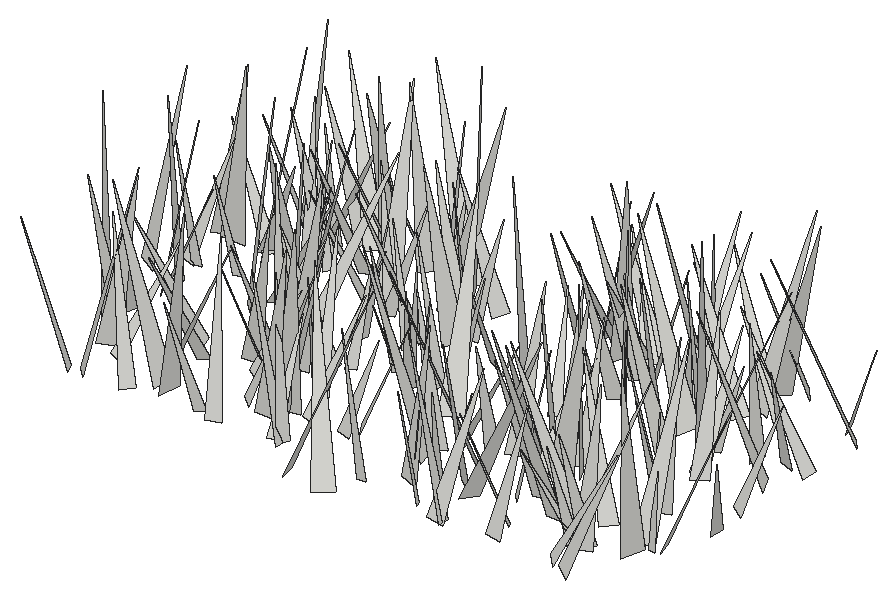
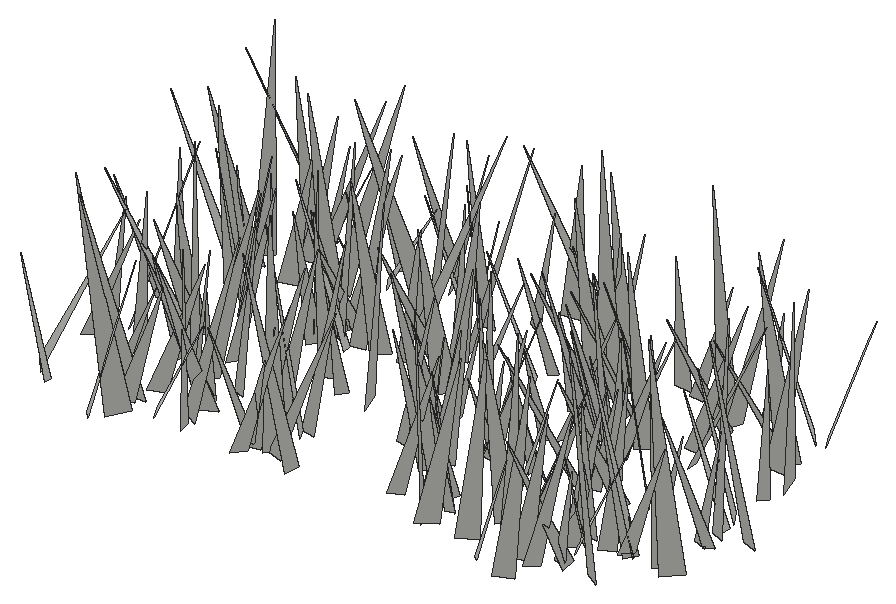
# SketchUp Ruby script. Lengths in inches.
U = 1.inch
M = Sketchup.active_model
def pt(a) = Geom::Point3d.new(a.map { |v| v * U })
def face(e, loops, mat)
  f = e.add_face(loops[0].map { |a| pt(a) })
  loops[1..].each { |l| e.add_face(l.map { |a| pt(a) }).erase! }
  f.material = f.back_material = mat if mat
  f
end
# faces: each face lists its corners as indices into pts; further lists are holes
def faces(e, pts, list, mat = nil) = list.each { |f| face(e, (f[0].is_a?(Array) ? f : [f]).map { |l| l.map { |i| pts[i] } }, mat) }
# xy, xz, yz: faces in a plane at the given z, y or x. An outline is a flat list of corners, or four numbers for a rectangle; further outlines are holes
def ring(l) = l.size == 4 ? [[l[0], l[1]], [l[2], l[1]], [l[2], l[3]], [l[0], l[3]]] : l.each_slice(2).to_a
def flat(e, list, mat, &to3) = list.each { |f| face(e, (f[0].is_a?(Array) ? f : [f]).map { |l| ring(l).map { |u, v| to3.(u, v) } }, mat) }
def xy(e, z, list, mat = nil) = flat(e, list, mat) { |x, y| [x, y, z] }
def xz(e, y, list, mat = nil) = flat(e, list, mat) { |x, z| [x, y, z] }
def yz(e, x, list, mat = nil) = flat(e, list, mat) { |y, z| [x, y, z] }
def lines(e, pts, list) = list.each { |a, b| e.add_line(pt(pts[a]), pt(pts[b])) }
# prism: a flat outline (further loops are holes) pulled along v
def prism(e, loops, v, mat = nil)
  f = face(e, loops, mat); d = Geom::Vector3d.new(v.map { |x| x * U })
  f.pushpull(f.normal.samedirection?(d) ? d.length : -d.length)
end
def box(e, o, s, mat = nil) = prism(e, [[o, [o[0] + s[0], o[1], o[2]], [o[0] + s[0], o[1] + s[1], o[2]], [o[0], o[1] + s[1], o[2]]]], [0, 0, s[2]], mat)
def at(x, y, z, deg = 0) = Geom::Transformation.translation(pt([x, y, z])) * Geom::Transformation.rotation(ORIGIN, Z_AXIS, deg.degrees)
def axes(o, x, y, z) = Geom::Transformation.new([*x, 0, *y, 0, *z, 0, *pt(o).to_a, 1])
def part(name) = M.definitions.add(name)
# library, detail: a bought-in or finely detailed component or shape, given as its bounding box
def library(name, o, s) = part(name).tap { |d| box(d.entities, o, s) }
def detail(e, o, s) = box(e.add_group.entities, o, s)
def put(e, d, t, mat = nil) = e.add_instance(d, t).tap { |i| i.material = mat if mat }
def group(e, t, mat = nil) = e.add_group.tap { |g| g.transformation = t; g.material = mat if mat }.entities
root = M.entities
c1 = part("fur_instance\#9")
p = [[0.8125,0,1.79],[0.67,-0.02,1.48],[0,-0.11,0],[0,0.11,0]]
faces(c1.entities,p,[[0,1,2,3]])
put(root,c1,axes([525.83,104.71,-21.66],[-2.86004,7.00076,0.77945],[7.00763,2.7424,1.08181],[-0.71502,-1.12544,7.48466]))
put(root,c1,axes([522.47,105.28,-21.66],[7.12948,2.21776,0.41944],[2.17259,-7.11974,0.71624],[-0.61174,0.56098,7.43203]))
put(root,c1,axes([503.1,107.16,-21.66],[-4.74174,-2.50609,0.51828],[-2.55748,4.67952,-0.77105],[0.09149,0.92453,5.30754]))
put(root,c1,axes([533.8125,106.15,-21.66],[0.03547,5.69131,1.501],[5.73382,0.30561,-1.29426],[1.32938,-1.46999,5.5423]))
put(root,c1,axes([534.32,106.38,-21.66],[-6.24639,-1.28271,0.8155],[-1.43317,6.11916,-1.35263],[0.50635,1.49608,6.23162]))
put(root,c1,axes([513.14,108.02,-21.66],[0.25989,-4.12749,1.06746],[-4.12688,-0.51192,-0.97467],[-1.06982,0.97209,4.01917]))
put(root,c1,axes([538.07,106.8,-21.66],[0.29151,4.89673,1.62599],[5.06271,0.04273,-1.03633],[0.99541,-1.65136,4.79468]))
put(root,c1,axes([542.84,106.84,-21.66],[3.55975,3.91646,0.08522],[3.79537,-3.41954,-1.38552],[0.97011,-0.99289,5.10792]))
put(root,c1,axes([531.6,107.22,-21.66],[-3.37291,-1.64413,0.77782],[-1.79286,3.28135,-0.83849],[0.30629,1.10194,3.65741]))
put(root,c1,axes([509.95,108.84,-21.66],[7.47084,-2.00529,1.5784],[-1.88161,-7.62701,-0.78379],[-1.72397,-0.36551,7.69548]))
put(root,c1,axes([544.35,106.04,-21.66],[4.64022,6.0526,0.40907],[6.0581,-4.59639,-0.71102],[0.31728,-0.75645,7.59342]))
put(root,c1,axes([526.85,107.35,-21.66],[-2.00481,-4.221,2.16779],[-4.72189,1.54205,-1.3643],[-0.46899,2.51807,4.46932]))
put(root,c1,axes([542.77,109.58,-21.66],[-3.89152,-1.38284,0.09587],[-1.31779,3.77936,1.02238],[0.42995,-0.93252,4.00136]))
put(root,c1,axes([543.67,109.5625,-21.66],[3.33283,-3.55166,1.19436],[-3.37517,-3.53973,-1.10774],[-1.62758,0.06765,4.74288]))
put(root,c1,axes([533.24,107.18,-21.66],[3.40494,2.47984,0.75094],[2.39973,-3.48584,0.63038],[-0.97714,0.08048,4.16483]))
put(root,c1,axes([542.47,109.48,-21.66],[-3.58815,0.95471,1.93369],[1.59157,3.70529,1.12394],[1.45517,-1.69849,3.5388]))
put(root,c1,axes([519.88,107.92,-21.66],[-5.84783,-0.54956,0.92386],[-0.66437,5.86496,-0.71656],[0.84507,0.80798,5.82972]))
put(root,c1,axes([537.84,108.75,-21.66],[-3.22375,-2.36609,0.00506],[-2.25529,3.0702,-1.21594],[-0.71558,0.9831,3.80952]))
put(root,c1,axes([529.29,109.17,-21.66],[-0.7765,-5.95979,2.50914],[-6.25232,1.3369,1.24057],[1.65027,2.26084,5.88073]))
put(root,c1,axes([509.01,109.41,-21.66],[-7.26017,0.65472,1.63239],[0.85,7.37598,0.82207],[1.53976,-0.9847,7.24313]))
put(root,c1,axes([507.7,107.36,-21.66],[-5.44212,1.96061,0.21811],[1.90755,5.39324,-0.88463],[0.50284,0.7598,5.71648]))
put(root,c1,axes([519.85,108.06,-21.66],[-5.54219,0.95074,1.40051],[0.80502,5.69802,-0.68242],[1.48905,0.4581,5.58158]))
put(root,c1,axes([514.65,107.5,-21.66],[-0.46142,6.00885,1.03301],[6.04976,0.32253,0.82618],[-0.75742,-1.08443,5.96964]))
put(root,c1,axes([543.51,109.09,-21.66],[3.4619,-5.09824,2.22403],[-5.52391,-3.4582,0.67108],[-0.65172,2.22978,6.12588]))
put(root,c1,axes([546.36,110.7,-21.66],[6.94101,-3.43299,1.84422],[-3.2352,-7.17632,-1.18245],[-2.17258,-0.28153,7.65277]))
put(root,c1,axes([516.83,110.11,-21.66],[2.07554,-6.96607,1.71735],[-7.11885,-1.77704,1.39545],[0.89291,2.02467,7.13349]))
put(root,c1,axes([532.55,110.9,-21.66],[-2.91514,-5.53327,1.42514],[-5.42873,3.18122,1.24695],[1.78243,0.63944,6.12864]))
put(root,c1,axes([530.92,110.16,-21.66],[3.87563,-0.57439,1.14349],[-0.32332,-3.96837,-0.89752],[-1.23813,-0.76168,3.81378]))
put(root,c1,axes([504.06,107.25,-21.66],[5.15399,5.0376,1.12923],[4.93282,-5.27609,1.02292],[-1.5231,-0.04087,7.13405]))
put(root,c1,axes([519.14,108.05,-21.66],[-2.23012,3.65012,0.738],[3.54975,2.34365,-0.86487],[1.12574,-0.15918,4.18913]))
put(root,c1,axes([539.7,111.2,-21.66],[-1.24664,-7.42641,1.30497],[-7.49381,1.07378,-1.04811],[-0.83512,1.45053,7.45702]))
put(root,c1,axes([542.29,110.39,-21.66],[-7.15146,0.58689,0.88826],[0.71619,7.11549,1.06478],[0.78773,-1.14116,7.09606]))
put(root,c1,axes([533.6,109.96,-21.66],[7.07032,-2.50038,0.22823],[-2.5064,-6.98854,1.08245],[0.14815,1.09629,7.42089]))
put(root,c1,axes([517.47,111.4375,-21.66],[3.37968,-7.43588,1.46776],[-7.57694,-3.27406,0.85991],[0.19143,1.6903,8.12251]))
put(root,c1,axes([503.16,111.08,-21.66],[4.2743,-5.66959,1.70794],[-5.91958,-4.14155,1.06631],[-0.14077,2.00854,7.01974]))
put(root,c1,axes([503.41,112.21,-21.66],[0.65749,-6.30029,1.7132],[-6.47052,-0.85883,-0.67511],[-0.87239,1.62165,6.29842]))
put(root,c1,axes([514.63,110.91,-21.66],[2.82445,3.52777,0.66946],[3.53756,-2.58781,-1.2883],[0.61561,-1.31488,4.33162]))
put(root,c1,axes([531.93,113.11,-21.66],[-4.63636,-6.55031,0.51962],[-6.56307,4.58532,-0.75728],[-0.32055,0.86066,7.9893]))
put(root,c1,axes([509.1,113.46,-21.66],[0.9036,-5.03288,0.01557],[-4.93923,-0.88981,-0.97923],[-0.96652,-0.158,5.01871]))
put(root,c1,axes([528.16,112.43,-21.66],[-7.66466,-1.90179,1.421],[-1.79066,7.78455,0.75987],[1.55871,-0.40873,7.86043]))
put(root,c1,axes([537.15,112.77,-21.66],[-0.33805,-5.61743,0.95415],[-5.65981,0.22074,-0.70569],[-0.6576,0.9879,5.58317]))
put(root,c1,axes([522.22,111.29,-21.66],[0.51441,-3.71167,1.78135],[-3.92489,0.09986,1.3415],[1.24297,1.85145,3.49879]))
put(root,c1,axes([504.625,110.06,-21.66],[1.15422,4.7345,0.08294],[4.6056,-1.10261,-1.15208],[1.10037,-0.35121,4.73502]))
put(root,c1,axes([508.52,110.51,-21.66],[4.79219,0.94532,0.41054],[0.81575,-4.67249,1.23678],[-0.62985,1.14081,4.72537]))
put(root,c1,axes([517.87,110.53,-21.66],[5.65388,1.0827,1.74004],[0.6959,-5.81697,1.3583],[-1.92762,1.07564,5.59407]))
put(root,c1,axes([527.24,112.375,-21.66],[4.80931,3.10321,2.02961],[3.46778,-4.94111,-0.66234],[-1.31293,-1.68352,5.68513]))
put(root,c1,axes([547.49,112.59,-21.66],[5.84375,1.80801,0.13219],[1.81029,-5.79638,-0.74876],[0.09603,-0.75425,6.07105]))
put(root,c1,axes([519.3,111.38,-21.66],[0.97735,4.73028,0.44464],[4.65378,-0.86171,-1.06216],[0.95682,-0.64061,4.71196]))
put(root,c1,axes([522.7,112.51,-21.66],[4.03846,2.29721,0.25382],[2.30928,-3.98992,-0.63131],[0.09403,-0.6739,4.60302]))
put(root,c1,axes([547.07,111.78,-21.66],[1.77865,4.09096,1.0407],[3.89915,-2.02489,1.29578],[-1.61729,-0.38272,4.26855]))
put(root,c1,axes([536.0625,111.66,-21.66],[3.62964,3.56201,0.97293],[3.43547,-3.75775,0.94107],[-1.35352,0.01415,4.99765]))
put(root,c1,axes([528.16,113.54,-21.66],[1.39978,-5.30319,2.32473],[-5.64349,-1.78474,-0.67328],[-1.29585,2.04412,5.44334]))
put(root,c1,axes([542.875,112.61,-21.66],[-3.19469,4.99874,1.10839],[5.10889,3.02549,1.08057],[-0.33936,-1.5103,5.83317]))
put(root,c1,axes([507.88,115.08,-21.66],[-5.4355,-1.48683,0.1699],[-1.41481,5.31415,1.24191],[0.48767,-1.15472,5.49664]))
put(root,c1,axes([534.19,116.32,-21.66],[-0.43827,-6.52973,0.002],[-6.42899,0.43186,1.145],[1.14256,-0.07472,6.44348]))
put(root,c1,axes([513.7,114.24,-21.66],[-2.53875,-3.10556,0.31926],[-3.0835,2.42999,-0.88252],[-0.48832,0.80145,3.91291]))
put(root,c1,axes([546.03,112.22,-21.66],[-1.91497,6.86191,1.78883],[6.91485,2.21764,-1.10438],[1.57179,-1.39609,7.03799]))
put(root,c1,axes([511.66,115.16,-21.66],[2.30675,-6.01681,0.97122],[-6.03702,-2.11321,1.24701],[0.83643,1.34116,6.32203]))
put(root,c1,axes([515.02,112.92,-21.66],[4.28943,0.41298,0.87796],[0.18379,-4.25331,1.1028],[-0.95267,1.03894,4.16576]))
put(root,c1,axes([501.53,115.66,-21.66],[3.7269,-2.05729,0.24824],[-1.97365,-3.67974,-0.86491],[-0.63149,-0.64103,4.16823]))
put(root,c1,axes([501.33,113.27,-21.66],[-7.33304,-1.55705,2.53328],[-2.07568,7.50758,-1.39398],[2.1292,1.95633,7.36578]))
put(root,c1,axes([536.71,115.34,-21.66],[-1.94061,6.26278,4.61542],[7.19839,3.24975,-1.38302],[2.95087,-3.80883,6.40903]))
put(root,c1,axes([548.84,116.17,-21.66],[3.9114,-1.46291,0.01114],[-1.40736,-3.77134,-1.11157],[-0.39945,-1.03737,4.02536]))
put(root,c1,axes([516.36,115.63,-21.66],[2.79226,2.81825,2.22878],[3.51982,-2.71249,-0.9798],[-0.72174,-2.32521,3.84438]))
put(root,c1,axes([525.09,115.17,-21.66],[-2.96371,-3.18096,0.56073],[-3.21747,2.84043,-0.89238],[-0.28422,1.01488,4.25508]))
put(root,c1,axes([530.68,115.92,-21.66],[2.96444,-3.24193,0.90441],[-3.19075,-3.09049,-0.61962],[-1.07107,0.23387,4.34903]))
put(root,c1,axes([512.91,113.75,-21.66],[2.64419,5.03318,0.33977],[4.95036,-2.51506,-1.26831],[0.97076,-0.88412,5.54221]))
put(root,c1,axes([514.43,116.13,-21.66],[3.42079,-7.2545,1.9343],[-7.49487,-3.17419,1.34998],[0.44283,2.31686,7.90614]))
put(root,c1,axes([535.65,116.32,-21.66],[3.71105,4.69804,3.51461],[5.68502,-3.90755,-0.77947],[-1.45074,-3.29476,5.93598]))
put(root,c1,axes([529.1,114.6,-21.66],[4.45979,0.0367,0.09292],[0.01604,-4.35825,0.95137],[-0.0986,0.95079,4.35729]))
put(root,c1,axes([544.46,115.97,-21.66],[3.53738,-5.32848,1.99163],[-5.66565,-3.51029,0.67133],[-0.50966,2.039,6.36044]))
put(root,c1,axes([512.27,116.77,-21.66],[-0.63614,-4.28295,0.71253],[-4.25699,0.4736,-0.95381],[-0.85404,0.8295,4.22357]))
put(root,c1,axes([536.11,115.47,-21.66],[4.52049,-0.19473,1.20973],[-0.39564,-4.60837,0.73662],[-1.15967,0.81315,4.46432]))
put(root,c1,axes([535.64,114.41,-21.66],[-1.08496,4.24211,0.2137],[4.12597,1.10497,-0.98676],[1.00871,0.04308,4.26602]))
put(root,c1,axes([517.94,114.35,-21.66],[-0.8094,5.47668,0.09308],[5.43232,0.79056,0.72297],[-0.70181,-0.19701,5.48875]))
put(root,c1,axes([534.66,116.9,-21.66],[5.44749,2.02001,0.26599],[2.02291,-5.27178,-1.39377],[0.24298,-1.39796,5.64031]))
put(root,c1,axes([542.72,117.6,-21.66],[3.69815,0.46024,1.83595],[1.02421,-3.87534,-1.09159],[-1.5917,-1.42435,3.56322]))
put(root,c1,axes([532.54,116.07,-21.66],[-2.8521,5.31504,2.52319],[5.50682,3.39878,-0.93481],[2.07151,-1.71732,5.95905]))
put(root,c1,axes([542.52,118.02,-21.66],[-4.88015,-2.78524,1.52655],[-2.68194,5.11285,0.7548],[1.7015,0.07051,5.5681]))
put(root,c1,axes([544.2,115.77,-21.66],[4.62309,3.63215,1.82021],[3.50208,-4.96051,1.00367],[-2.05939,-0.28182,5.79293]))
put(root,c1,axes([516.47,117.65,-21.66],[-5.33847,-0.05884,0.40473],[-0.0096,5.31499,0.64603],[0.40887,-0.64342,5.29956]))
put(root,c1,axes([521.91,118.4,-21.66],[4.60045,-1.39498,0.802],[-1.20201,-4.59424,-1.0961],[-1.06973,-0.83684,4.68067]))
put(root,c1,axes([537.4,116.625,-21.66],[-5.47988,-2.79163,2.54101],[-3.31815,5.69792,-0.89593],[1.79996,2.00489,6.08438]))
put(root,c1,axes([539.3,118.63,-21.66],[4.52719,2.71843,2.25301],[3.1828,-4.72799,-0.69084],[-1.52829,-1.79378,5.23527]))
put(root,c1,axes([513,117.35,-21.66],[-6.34859,-2.07949,3.15929],[-2.7531,6.77324,-1.07409],[2.59343,2.09974,6.59357]))
put(root,c1,axes([512.7,117.11,-21.66],[5.61181,2.09612,1.30854],[1.89864,-5.73587,1.04566],[-1.58152,0.55181,5.89854]))
put(root,c1,axes([536.69,117.59,-21.66],[3.58302,-2.92408,2.58959],[-3.63927,-3.77537,0.77237],[-1.41842,2.30013,4.5598]))
put(root,c1,axes([514.33,116.67,-21.66],[2.31766,5.02687,0.82298],[4.84651,-2.45447,1.34356],[-1.56781,-0.15629,5.3699]))
put(root,c1,axes([512.23,117.46,-21.66],[-5.96382,1.04535,0.88629],[0.82737,5.90096,-1.39268],[1.09259,1.23747,5.8924]))
put(root,c1,axes([517.27,118.26,-21.66],[-2.50227,2.59124,1.1484],[2.47228,2.74461,-0.80603],[1.38608,-0.21748,3.51087]))
put(root,c1,axes([521,119.76,-21.66],[-1.15878,-4.12917,1.68532],[-4.31214,1.48176,0.66553],[1.13832,1.40977,4.23673]))
put(root,c1,axes([548.17,119.15,-21.66],[1.81296,4.05322,0.9149],[4.0683,-1.5284,-1.29051],[0.84535,-1.3371,4.24853]))
put(root,c1,axes([519.85,119.73,-21.66],[-1.05409,-4.02831,1.60299],[-4.27873,0.70037,-1.05356],[-0.69957,1.78611,4.02845]))
put(root,c1,axes([526.15,117.43,-21.66],[-5.32969,5.59283,1.04722],[5.46672,5.43108,-1.18331],[1.57839,0.07463,7.63447]))
put(root,c1,axes([500.93,120.21,-21.66],[4.64757,1.11707,0.03174],[1.0994,-4.54603,-0.98676],[0.20042,-0.96672,4.67697]))
put(root,c1,axes([501.52,118.66,-21.66],[-4.45958,-2.36263,3.46386],[-3.3219,5.07642,-0.81428],[2.55838,2.47306,4.98064]))
put(root,c1,axes([500.88,121.2,-21.66],[-3.13728,-6.42445,2.27927],[-6.51063,3.56742,1.09378],[2.01998,1.52023,7.06539]))
put(root,c1,axes([533.22,120.59,-21.66],[1.79677,-5.19077,1.98742],[-5.55817,-1.66844,0.66734],[0.02536,2.09632,5.45226]))
put(root,c1,axes([512.23,119.02,-21.66],[7.1658,2.76652,1.69463],[2.58302,-7.35112,1.0785],[-1.96302,0.42601,7.60521]))
put(root,c1,axes([510.76,121.36,-21.66],[1.65267,-3.08975,1.39314],[-3.11179,-1.99748,-0.7386],[-1.34319,0.82596,3.42525]))
put(root,c1,axes([523.22,119.97,-21.66],[-5.0928,-0.09663,0.30052],[-0.16718,4.94609,-1.24277],[0.26777,1.25023,4.93978]))
put(root,c1,axes([547.4375,122.9375,-21.66],[-6.20771,-3.16783,0.82777],[-3.08728,6.25411,0.78157],[1.09042,-0.32718,6.92531]))
put(root,c1,axes([524.13,120.52,-21.66],[3.78689,-0.0231,1.24793],[-0.32688,-3.86581,0.92039],[-1.20458,0.97644,3.67342]))
put(root,c1,axes([498.52,120.87,-21.66],[3.30058,6.51639,2.13105],[6.85171,-3.21879,-0.76942],[-0.24255,-2.25268,7.26396]))
put(root,c1,axes([539.24,122.68,-21.66],[-6.05597,0.77226,2.0179],[1.21073,6.18666,1.26588],[1.78953,-1.57224,5.97233]))
put(root,c1,axes([507.14,120.44,-21.66],[4.85297,5.01471,2.08252],[4.89411,-5.24941,1.23566],[-2.35199,-0.5761,6.86817]))
put(root,c1,axes([529.1,121.48,-21.66],[-7.32615,-2.19993,2.60741],[-2.57876,7.61493,-0.82074],[2.23345,1.57604,7.60517]))
put(root,c1,axes([543.68,120.91,-21.66],[3.74309,-3.05687,3.19875],[-4.02453,-4.09315,0.7978],[-1.83838,2.73658,4.76642]))
put(root,c1,axes([514.06,122.37,-21.66],[2.61371,2.45973,0.53308],[2.49517,-2.43181,-1.01309],[0.32949,-1.09634,3.44317]))
put(root,c1,axes([524.23,124.29,-21.66],[-1.58112,-4.73276,0.31075],[-4.65779,1.61119,0.83937],[0.89473,0.02406,4.91878]))
put(root,c1,axes([515.36,121.86,-21.66],[4.20313,-0.16718,1.34956],[-0.39887,-4.34286,0.70427],[-1.30006,0.79192,4.14708]))
put(root,c1,axes([501.12,122.7,-21.66],[-0.94166,-4.10224,1.61468],[-4.38512,0.70145,-0.77524],[-0.45421,1.73259,4.13692]))
put(root,c1,axes([518.23,124.21,-21.66],[-5.1626,-2.88411,0.4563],[-2.82641,5.16852,0.6903],[0.7333,-0.3834,5.87316]))
put(root,c1,axes([507.92,122.01,-21.66],[4.70172,-1.10111,0.26171],[-1.12934,-4.49092,1.39405],[0.07438,1.41645,4.62334]))
put(root,c1,axes([503.99,123.31,-21.66],[-0.09942,-3.58739,1.13729],[-3.70553,-0.10534,-0.65623],[-0.65715,1.13676,3.52826]))
put(root,c1,axes([518.55,122.47,-21.66],[-0.54656,4.2534,1.19948],[4.32093,0.26075,1.04426],[-0.92722,-1.29209,4.15928]))
put(root,c1,axes([531.24,121.64,-21.66],[-2.96108,3.10315,0.36366],[3.04624,2.97875,-0.6142],[0.69442,0.16515,4.24503]))
put(root,c1,axes([543.19,121.43,-21.66],[-2.46279,4.53865,0.90199],[4.34757,2.61941,-1.3098],[1.58479,-0.13272,4.99491]))
put(root,c1,axes([500.37,122.74,-21.66],[0.61438,4.77457,1.24038],[4.786,-0.27399,-1.3159],[1.1955,-1.35681,4.63059]))
put(root,c1,axes([520.41,124.86,-21.66],[4.49335,-4.83843,2.48866],[-4.8443,-5.0271,-1.02712],[-2.47721,1.05444,6.5227]))
put(root,c1,axes([511.64,121.79,-21.66],[1.69788,6.23349,0.03172],[6.16311,-1.67374,-0.97718],[0.93461,-0.28707,6.38626]))
put(root,c1,axes([546.875,125.73,-21.66],[-0.66532,-4.77379,0.4836],[-4.67341,0.75535,1.0268],[1.0873,0.32553,4.70929]))
put(root,c1,axes([542.84,122.4,-21.66],[6.48449,2.8801,0.19854],[2.8437,-6.45643,0.78158],[-0.49773,0.63448,7.05214]))
put(root,c1,axes([536.36,125.76,-21.66],[-2.50316,-5.2047,1.47138],[-5.2002,2.76171,0.92225],[1.48721,0.89649,5.70124]))
put(root,c1,axes([532.87,125.8125,-21.66],[1.51569,-5.39227,1.25729],[-5.41404,-1.71643,-0.83467],[-1.15995,0.96539,5.5387]))
put(root,c1,axes([544.9375,125.22,-21.66],[-4.81176,0.83188,2.6308],[1.27412,5.3609,0.63523],[2.44739,-1.15538,4.84165]))
put(root,c1,axes([542.14,124.41,-21.66],[2.6099,-2.39325,0.8726],[-2.54736,-2.4537,0.88934],[-0.00348,1.24593,3.42758]))
put(root,c1,axes([512.07,126.12,-21.66],[-4.07436,-2.22938,0.28557],[-2.14023,4.02883,0.91657],[0.68639,-0.67121,4.55307]))
put(root,c1,axes([539.99,125.67,-21.66],[7.38345,1.68053,2.79244],[2.22073,-7.65548,-1.26461],[-2.38543,-1.92527,7.46594]))
put(root,c1,axes([548.79,125.73,-21.66],[-4.51725,1.3418,0.80765],[1.52463,4.33149,1.33117],[0.35811,-1.51528,4.52039]))
put(root,c1,axes([529.7,127.03,-21.66],[-1.86711,-6.21996,0.83765],[-6.21183,1.95621,0.67975],[0.89595,0.60083,6.45848]))
put(root,c1,axes([505.19,127.04,-21.66],[4.3108,-3.69492,0.61953],[-3.55093,-4.33068,-1.12044],[-1.19463,-0.46051,5.56597]))
put(root,c1,axes([539.13,125.43,-21.66],[-7.00283,2.97011,1.6591],[3.21934,7.01289,1.03394],[1.10002,-1.61605,7.53606]))
put(root,c1,axes([500.92,126.63,-21.66],[1.84601,-7.44066,1.73932],[-7.59322,-1.58595,1.27441],[0.85535,1.97933,7.55956]))
put(root,c1,axes([499.92,127.03,-21.66],[4.60789,-6.31495,1.14074],[-6.41656,-4.51508,0.92427],[0.08686,1.46561,7.76253]))
put(root,c1,axes([534.02,125.18,-21.66],[3.38997,4.6985,2.258],[4.82742,-3.84601,0.75539],[-1.96736,-1.34115,5.74432]))
put(root,c1,axes([514.75,125.18,-21.66],[3.82826,-1.89723,1.31218],[-2.241,-3.66166,1.2438],[-0.54703,1.72325,4.08754]))
put(root,c1,axes([503.53,126.77,-21.66],[3.31192,-3.28223,0.0309],[-3.2384,-3.26025,0.79144],[0.53549,0.5836,4.59516]))
put(root,c1,axes([520.81,126.02,-21.66],[1.98838,-4.24744,1.75797],[-4.57109,-1.62434,1.24561],[0.4862,2.09896,4.52138]))
put(root,c1,axes([520.7,125.84,-21.66],[-4.62696,-2.40171,1.71965],[-2.7299,4.69747,-0.78458],[1.12828,1.51649,5.15378]))
put(root,c1,axes([539.83,125.88,-21.66],[-4.89428,-1.48699,1.50253],[-1.73277,4.99254,-0.70337],[1.21087,1.13406,5.0666]))
put(root,c1,axes([537.2,127.65,-21.66],[0.94706,-3.59902,0.23008],[-3.53322,-0.8783,0.80484],[0.72266,0.42244,3.63347]))
put(root,c1,axes([519.43,126.89,-21.66],[-4.54367,3.48057,1.82928],[3.81076,4.58683,0.73803],[0.96889,-1.71821,5.67579]))
put(root,c1,axes([503.85,126.81,-21.66],[-3.48001,3.233,0.8636],[3.33945,3.27515,1.19585],[-0.21495,-1.45934,4.59703]))
put(root,c1,axes([529.92,127.42,-21.66],[6.22111,3.48137,1.76986],[3.77865,-6.20685,-1.07301],[-0.98698,-1.81924,7.04775]))
put(root,c1,axes([510.18,128.58,-21.66],[-0.32554,-5.06602,0.7464],[-4.99056,0.14633,-1.18345],[-1.14716,0.80105,4.9366]))
put(root,c1,axes([513.71,126.72,-21.66],[-0.78367,4.54033,1.31363],[4.69244,0.5877,0.76808],[-0.56674,-1.41222,4.54299]))
put(root,c1,axes([503.8,126.04,-21.66],[6.26441,4.08516,1.86388],[4.05019,-6.52197,0.68206],[-1.9387,-0.42509,7.44756]))
put(root,c1,axes([507.48,128.11,-21.66],[-4.95355,2.49117,1.9463],[2.93301,4.97148,1.10159],[1.17959,-1.90003,5.43416]))
put(root,c1,axes([507.28,126.39,-21.66],[-0.20928,5.81187,1.2771],[5.90875,0.05179,0.73257],[-0.70395,-1.2931,5.76932]))
put(root,c1,axes([532.45,128.65,-21.66],[0.82361,-5.861,1.93807],[-5.93962,-1.28507,-1.3621],[-1.68178,1.66825,5.75972]))
put(root,c1,axes([506.9,128.0625,-21.66],[-4.69197,-2.31538,0.05263],[-2.28134,4.60011,-1.00642],[-0.39908,0.92541,5.13447]))
put(root,c1,axes([508.08,127.42,-21.66],[-3.93894,0.78438,0.2139],[0.7314,3.88076,-0.76228],[0.35506,0.70765,3.94328]))
put(root,c1,axes([531.32,130.67,-21.66],[3.03189,-3.59681,0.02756],[-3.43565,-2.90654,-1.37057],[-1.06494,-0.8632,4.50011]))
put(root,c1,axes([510.91,130.9,-21.66],[-3.83453,-4.44323,0.31037],[-4.29048,3.7947,1.3169],[1.19597,-0.63261,5.71941]))
put(root,c1,axes([506.93,127.31,-21.66],[2.12896,3.50938,0.78952],[3.35263,-2.26833,1.04217],[-1.30344,-0.10245,3.97015]))
put(root,c1,axes([533.06,128.55,-21.66],[0.75971,3.71481,1.88794],[3.89435,-1.31575,1.02184],[-1.48263,-1.55251,3.65142]))
put(root,c1,axes([517.31,128.3125,-21.66],[7.2049,-3.47591,1.96261],[-3.83046,-7.15988,1.38131],[-1.1231,2.12096,7.87937]))
put(root,c1,axes([529.9,130.19,-21.66],[6.97183,-3.45055,1.53762],[-3.37643,-7.13932,-0.71191],[-1.69419,0.0288,7.74635]))
put(root,c1,axes([529.5,130.66,-21.66],[-1.20375,-5.21342,0.24756],[-5.17288,1.15789,-0.76855],[-0.69453,0.4118,5.2951]))
put(root,c1,axes([540.64,128.77,-21.66],[-4.45803,3.98436,0.74293],[4.03358,4.25341,1.39275],[-0.39655,-1.52789,5.81458]))
put(root,c1,axes([520.36,129.69,-21.66],[-4.35819,2.96505,1.59627],[3.3258,4.19926,1.28011],[0.52792,-1.97688,5.11338]))
put(root,c1,axes([512.49,128.2,-21.66],[-3.77046,5.93467,2.17976],[6.06315,4.1134,-0.71146],[1.79161,-1.43096,6.99504]))
put(root,c1,axes([536.93,130.14,-21.66],[-2.90211,-6.23156,1.67253],[-6.44447,2.71044,-1.08359],[-0.31368,1.96803,6.78825]))
put(root,c1,axes([543.29,129.8,-21.66],[-3.79672,1.89832,0.59417],[1.98792,3.66583,0.99077],[0.06937,-1.15319,4.1276]))
put(root,c1,axes([537.78,127.36,-21.66],[0.187,6.43803,0.46404],[6.40843,-0.12967,-0.78342],[0.77175,-0.48321,6.39292]))
put(root,c1,axes([516.23,129.34,-21.66],[0.00091,-3.67707,1.93886],[-4.08733,0.35251,0.67045],[0.75747,1.90654,3.61543]))
put(root,c1,axes([548.65,130.72,-21.66],[-5.4011,-4.4458,0.12135],[-4.40164,5.31613,-1.14717],[-0.63674,0.96192,6.9008]))
put(root,c1,axes([533.65,128.59,-21.66],[3.84083,1.33111,0.88578],[1.09907,-3.87194,1.0529],[-1.16125,0.73803,3.92622]))
put(root,c1,axes([510.02,131.18,-21.66],[-0.4517,-7.27096,2.0225],[-7.50286,0.65147,0.6664],[0.81515,1.96726,7.25444]))
put(root,c1,axes([516.55,128.7,-21.66],[3.29752,4.92899,1.52703],[4.76096,-3.60504,1.35547],[-1.98997,-0.45731,5.77332]))
put(root,c1,axes([503.68,130.51,-21.66],[4.80804,6.17674,2.98381],[6.78482,-4.81897,-0.95722],[-1.01068,-2.96612,7.76873]))
put(root,c1,axes([536.38,131.29,-21.66],[5.52429,1.58059,2.16664],[1.98524,-5.74559,-0.8703],[-1.80317,-1.48335,5.67966]))
put(root,c1,axes([527.5,131.46,-21.66],[7.30646,0.41261,0.41525],[0.46932,-7.23653,-1.06747],[-0.34987,-1.09065,7.23983]))
put(root,c1,axes([536.5,128.67,-21.66],[-1.23708,6.4323,0.84499],[6.38548,1.35924,-0.99849],[1.14637,-0.62994,6.47363]))
put(root,c1,axes([513.18,131.36,-21.66],[3.99451,-5.40043,2.70776],[-5.64329,-4.49426,-0.63847],[-2.15638,1.75774,6.68679]))
put(root,c1,axes([506.53,130.25,-21.66],[0.17252,3.92598,1.26935],[3.97591,-0.49782,0.99933],[-1.10305,-1.18034,3.80058]))
put(root,c1,axes([507.77,131.55,-21.66],[-5.02237,2.51021,1.68016],[2.86774,4.98644,1.12241],[0.94877,-1.78398,5.50142]))
put(root,c1,axes([539.04,130.91,-21.66],[-4.27231,-1.94809,0.06255],[-1.87913,4.07681,-1.37844],[-0.51754,1.27912,4.48861]))
put(root,c1,axes([505.97,130.08,-21.66],[4.9565,-0.0282,0.53243],[-0.1703,-4.80111,1.33099],[-0.50525,1.34155,4.77453]))
put(root,c1,axes([547,131.99,-21.66],[4.10425,1.09153,0.3293],[1.14011,-3.92312,-1.20584],[0.00571,-1.24998,4.07214]))
put(root,c1,axes([541.01,130.31,-21.66],[1.96643,7.28816,1.86053],[7.47956,-1.69089,-1.28167],[0.79683,-2.11408,7.43918]))
put(root,c1,axes([511.16,133.04,-21.66],[-2.38013,-2.88459,0.25848],[-2.75196,2.35686,0.96161],[0.90246,-0.42079,3.61403]))
put(root,c1,axes([517.23,130.96,-21.66],[6.18055,4.14964,3.19418],[4.26505,-6.85588,0.65402],[-3.03836,-1.18276,7.41558]))
put(root,c1,axes([541.47,131,-21.66],[-3.45745,4.3845,0.64107],[4.38114,3.2607,1.32749],[-0.66366,-1.31634,5.42361]))
put(root,c1,axes([540.75,132.62,-21.66],[6.79044,-4.4332,0.71146],[-4.48312,-6.76549,0.63187],[-0.24718,0.91888,8.0848]))
put(root,c1,axes([531.81,130.73,-21.66],[-2.66965,3.73747,0.14274],[3.69986,2.61324,0.77338],[-0.54785,-0.56423,4.52743]))
put(root,c1,axes([531.67,131.64,-21.66],[-5.56985,2.38046,0.65327],[2.45077,5.52546,0.76123],[0.29505,-0.95874,6.00918]))
put(root,c1,axes([508.24,133.91,-21.66],[4.15376,-5.21591,0.7578],[-5.12927,-4.22232,-0.94677],[-1.21268,-0.00681,6.60024]))
put(root,c1,axes([542.1875,133.96,-21.66],[-3.97091,-3.72473,0.66515],[-3.58252,4.01146,1.07602],[1.21718,-0.34456,5.33703]))
put(root,c1,axes([508.82,131.36,-21.66],[-4.49285,4.90641,0.97236],[5.00159,4.41981,0.80831],[0.04935,-1.26349,6.60342]))
put(root,c1,axes([516.4375,131.46,-21.66],[-5.45873,5.352,1.02249],[5.44819,5.38274,0.9113],[0.08123,-1.36725,7.5902]))
